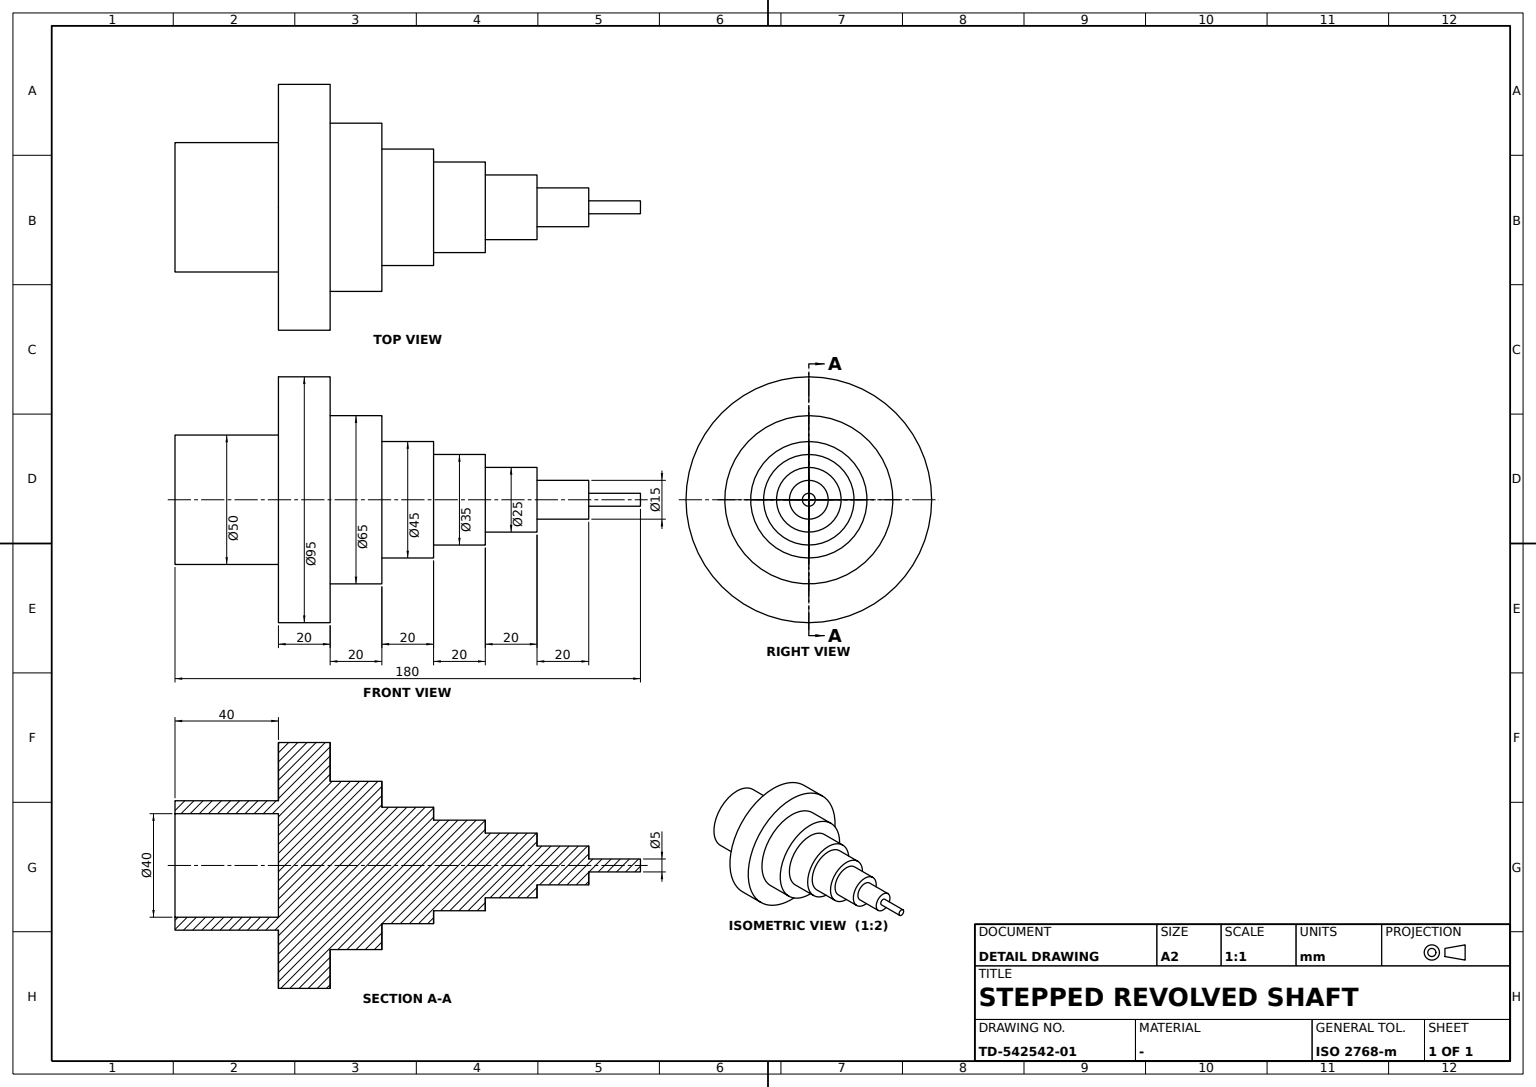
ISO-10303-21;
HEADER;
FILE_DESCRIPTION((''),'2;1');
FILE_NAME('','',(''),(''),'','','');
FILE_SCHEMA(('AUTOMOTIVE_DESIGN'));
ENDSEC;
DATA;
#1=APPLICATION_CONTEXT('');
#2=PRODUCT_CONTEXT('',#1,'mechanical');
#3=PRODUCT('','','',(#2));
#4=PRODUCT_DEFINITION_FORMATION('','',#3);
#5=PRODUCT_DEFINITION_CONTEXT('',#1,'design');
#6=PRODUCT_DEFINITION('','',#4,#5);
#7=PRODUCT_DEFINITION_SHAPE('','',#6);
#8=(LENGTH_UNIT()NAMED_UNIT(*)SI_UNIT(.MILLI.,.METRE.));
#9=(NAMED_UNIT(*)PLANE_ANGLE_UNIT()SI_UNIT($,.RADIAN.));
#10=(NAMED_UNIT(*)SI_UNIT($,.STERADIAN.)SOLID_ANGLE_UNIT());
#11=UNCERTAINTY_MEASURE_WITH_UNIT(LENGTH_MEASURE(0.005),#8,'distance_accuracy_value','');
#12=(GEOMETRIC_REPRESENTATION_CONTEXT(3)GLOBAL_UNCERTAINTY_ASSIGNED_CONTEXT((#11))GLOBAL_UNIT_ASSIGNED_CONTEXT((#8,#9,#10))REPRESENTATION_CONTEXT('',''));
#13=CARTESIAN_POINT('',(0.,140.,12.5));
#14=VERTEX_POINT('',#13);
#15=CARTESIAN_POINT('',(0.,140.,0.));
#16=DIRECTION('',(0.,1.,0.));
#17=DIRECTION('',(0.,0.,1.));
#18=AXIS2_PLACEMENT_3D('',#15,#16,#17);
#19=CIRCLE('',#18,12.5);
#20=EDGE_CURVE('',#14,#14,#19,.T.);
#21=ORIENTED_EDGE('',*,*,#20,.T.);
#22=EDGE_LOOP('',(#21));
#23=FACE_BOUND('',#22,.T.);
#24=CARTESIAN_POINT('',(0.,140.,7.5));
#25=VERTEX_POINT('',#24);
#26=CIRCLE('',#18,7.5);
#27=EDGE_CURVE('',#25,#25,#26,.T.);
#28=ORIENTED_EDGE('',*,*,#27,.F.);
#29=EDGE_LOOP('',(#28));
#30=FACE_BOUND('',#29,.T.);
#31=DIRECTION('',(1.,0.,0.));
#32=AXIS2_PLACEMENT_3D('',#13,#16,#31);
#33=PLANE('',#32);
#34=ADVANCED_FACE('',(#23,#30),#33,.T.);
#35=CARTESIAN_POINT('',(0.,40.,20.));
#36=VERTEX_POINT('',#35);
#37=CARTESIAN_POINT('',(0.,40.,0.));
#38=AXIS2_PLACEMENT_3D('',#37,#16,#17);
#39=CIRCLE('',#38,20.);
#40=EDGE_CURVE('',#36,#36,#39,.T.);
#41=ORIENTED_EDGE('',*,*,#40,.F.);
#42=EDGE_LOOP('',(#41));
#43=FACE_BOUND('',#42,.T.);
#44=CARTESIAN_POINT('',(0.,40.,25.));
#45=AXIS2_PLACEMENT_3D('',#44,#16,#31);
#46=PLANE('',#45);
#47=ADVANCED_FACE('',(#43),#46,.F.);
#48=CARTESIAN_POINT('',(0.,60.,32.5));
#49=VERTEX_POINT('',#48);
#50=CARTESIAN_POINT('',(0.,60.,0.));
#51=AXIS2_PLACEMENT_3D('',#50,#16,#17);
#52=CIRCLE('',#51,32.5);
#53=EDGE_CURVE('',#49,#49,#52,.T.);
#54=ORIENTED_EDGE('',*,*,#53,.F.);
#55=EDGE_LOOP('',(#54));
#56=FACE_BOUND('',#55,.T.);
#57=CARTESIAN_POINT('',(0.,60.,47.5));
#58=VERTEX_POINT('',#57);
#59=CIRCLE('',#51,47.5);
#60=EDGE_CURVE('',#58,#58,#59,.T.);
#61=ORIENTED_EDGE('',*,*,#60,.T.);
#62=EDGE_LOOP('',(#61));
#63=FACE_BOUND('',#62,.T.);
#64=AXIS2_PLACEMENT_3D('',#57,#16,#31);
#65=PLANE('',#64);
#66=ADVANCED_FACE('',(#56,#63),#65,.T.);
#67=CARTESIAN_POINT('',(0.,100.,17.5));
#68=VERTEX_POINT('',#67);
#69=CARTESIAN_POINT('',(0.,100.,0.));
#70=AXIS2_PLACEMENT_3D('',#69,#16,#17);
#71=CIRCLE('',#70,17.5);
#72=EDGE_CURVE('',#68,#68,#71,.T.);
#73=ORIENTED_EDGE('',*,*,#72,.T.);
#74=EDGE_LOOP('',(#73));
#75=FACE_BOUND('',#74,.T.);
#76=CARTESIAN_POINT('',(0.,120.,17.5));
#77=VERTEX_POINT('',#76);
#78=CARTESIAN_POINT('',(0.,120.,0.));
#79=AXIS2_PLACEMENT_3D('',#78,#16,#17);
#80=CIRCLE('',#79,17.5);
#81=EDGE_CURVE('',#77,#77,#80,.T.);
#82=ORIENTED_EDGE('',*,*,#81,.F.);
#83=EDGE_LOOP('',(#82));
#84=FACE_BOUND('',#83,.T.);
#85=CARTESIAN_POINT('',(0.,90.,0.));
#86=AXIS2_PLACEMENT_3D('',#85,#16,#31);
#87=CYLINDRICAL_SURFACE('',#86,17.5);
#88=ADVANCED_FACE('',(#75,#84),#87,.T.);
#89=ORIENTED_EDGE('',*,*,#60,.F.);
#90=EDGE_LOOP('',(#89));
#91=FACE_BOUND('',#90,.T.);
#92=CARTESIAN_POINT('',(0.,40.,47.5));
#93=VERTEX_POINT('',#92);
#94=CIRCLE('',#38,47.5);
#95=EDGE_CURVE('',#93,#93,#94,.T.);
#96=ORIENTED_EDGE('',*,*,#95,.T.);
#97=EDGE_LOOP('',(#96));
#98=FACE_BOUND('',#97,.T.);
#99=CYLINDRICAL_SURFACE('',#86,47.5);
#100=ADVANCED_FACE('',(#91,#98),#99,.T.);
#101=CARTESIAN_POINT('',(0.,100.,22.5));
#102=VERTEX_POINT('',#101);
#103=CIRCLE('',#70,22.5);
#104=EDGE_CURVE('',#102,#102,#103,.T.);
#105=ORIENTED_EDGE('',*,*,#104,.T.);
#106=EDGE_LOOP('',(#105));
#107=FACE_BOUND('',#106,.T.);
#108=ORIENTED_EDGE('',*,*,#72,.F.);
#109=EDGE_LOOP('',(#108));
#110=FACE_BOUND('',#109,.T.);
#111=AXIS2_PLACEMENT_3D('',#101,#16,#31);
#112=PLANE('',#111);
#113=ADVANCED_FACE('',(#107,#110),#112,.T.);
#114=CARTESIAN_POINT('',(0.,120.,12.5));
#115=VERTEX_POINT('',#114);
#116=CIRCLE('',#79,12.5);
#117=EDGE_CURVE('',#115,#115,#116,.T.);
#118=ORIENTED_EDGE('',*,*,#117,.F.);
#119=EDGE_LOOP('',(#118));
#120=FACE_BOUND('',#119,.T.);
#121=ORIENTED_EDGE('',*,*,#81,.T.);
#122=EDGE_LOOP('',(#121));
#123=FACE_BOUND('',#122,.T.);
#124=AXIS2_PLACEMENT_3D('',#76,#16,#31);
#125=PLANE('',#124);
#126=ADVANCED_FACE('',(#120,#123),#125,.T.);
#127=CARTESIAN_POINT('',(0.,160.,2.5));
#128=VERTEX_POINT('',#127);
#129=CARTESIAN_POINT('',(0.,160.,0.));
#130=AXIS2_PLACEMENT_3D('',#129,#16,#17);
#131=CIRCLE('',#130,2.5);
#132=EDGE_CURVE('',#128,#128,#131,.T.);
#133=ORIENTED_EDGE('',*,*,#132,.T.);
#134=EDGE_LOOP('',(#133));
#135=FACE_BOUND('',#134,.T.);
#136=CARTESIAN_POINT('',(0.,180.,2.5));
#137=VERTEX_POINT('',#136);
#138=CARTESIAN_POINT('',(0.,180.,0.));
#139=AXIS2_PLACEMENT_3D('',#138,#16,#17);
#140=CIRCLE('',#139,2.5);
#141=EDGE_CURVE('',#137,#137,#140,.T.);
#142=ORIENTED_EDGE('',*,*,#141,.F.);
#143=EDGE_LOOP('',(#142));
#144=FACE_BOUND('',#143,.T.);
#145=CYLINDRICAL_SURFACE('',#86,2.5);
#146=ADVANCED_FACE('',(#135,#144),#145,.T.);
#147=CARTESIAN_POINT('',(0.,160.,7.5));
#148=VERTEX_POINT('',#147);
#149=CIRCLE('',#130,7.5);
#150=EDGE_CURVE('',#148,#148,#149,.T.);
#151=ORIENTED_EDGE('',*,*,#150,.F.);
#152=EDGE_LOOP('',(#151));
#153=FACE_BOUND('',#152,.T.);
#154=ORIENTED_EDGE('',*,*,#27,.T.);
#155=EDGE_LOOP('',(#154));
#156=FACE_BOUND('',#155,.T.);
#157=CYLINDRICAL_SURFACE('',#86,7.5);
#158=ADVANCED_FACE('',(#153,#156),#157,.T.);
#159=ORIENTED_EDGE('',*,*,#104,.F.);
#160=EDGE_LOOP('',(#159));
#161=FACE_BOUND('',#160,.T.);
#162=CARTESIAN_POINT('',(0.,80.,22.5));
#163=VERTEX_POINT('',#162);
#164=CARTESIAN_POINT('',(0.,80.,0.));
#165=AXIS2_PLACEMENT_3D('',#164,#16,#17);
#166=CIRCLE('',#165,22.5);
#167=EDGE_CURVE('',#163,#163,#166,.T.);
#168=ORIENTED_EDGE('',*,*,#167,.T.);
#169=EDGE_LOOP('',(#168));
#170=FACE_BOUND('',#169,.T.);
#171=CYLINDRICAL_SURFACE('',#86,22.5);
#172=ADVANCED_FACE('',(#161,#170),#171,.T.);
#173=CARTESIAN_POINT('',(0.,0.,20.));
#174=VERTEX_POINT('',#173);
#175=CARTESIAN_POINT('',(0.,0.,0.));
#176=AXIS2_PLACEMENT_3D('',#175,#16,#17);
#177=CIRCLE('',#176,20.);
#178=EDGE_CURVE('',#174,#174,#177,.T.);
#179=ORIENTED_EDGE('',*,*,#178,.F.);
#180=EDGE_LOOP('',(#179));
#181=FACE_BOUND('',#180,.T.);
#182=ORIENTED_EDGE('',*,*,#40,.T.);
#183=EDGE_LOOP('',(#182));
#184=FACE_BOUND('',#183,.T.);
#185=CARTESIAN_POINT('',(0.,0.1,0.));
#186=AXIS2_PLACEMENT_3D('',#185,#16,#31);
#187=CYLINDRICAL_SURFACE('',#186,20.);
#188=ADVANCED_FACE('',(#181,#184),#187,.F.);
#189=CARTESIAN_POINT('',(0.,80.,32.5));
#190=VERTEX_POINT('',#189);
#191=CIRCLE('',#165,32.5);
#192=EDGE_CURVE('',#190,#190,#191,.T.);
#193=ORIENTED_EDGE('',*,*,#192,.T.);
#194=EDGE_LOOP('',(#193));
#195=FACE_BOUND('',#194,.T.);
#196=ORIENTED_EDGE('',*,*,#167,.F.);
#197=EDGE_LOOP('',(#196));
#198=FACE_BOUND('',#197,.T.);
#199=AXIS2_PLACEMENT_3D('',#189,#16,#31);
#200=PLANE('',#199);
#201=ADVANCED_FACE('',(#195,#198),#200,.T.);
#202=ORIENTED_EDGE('',*,*,#192,.F.);
#203=EDGE_LOOP('',(#202));
#204=FACE_BOUND('',#203,.T.);
#205=ORIENTED_EDGE('',*,*,#53,.T.);
#206=EDGE_LOOP('',(#205));
#207=FACE_BOUND('',#206,.T.);
#208=CYLINDRICAL_SURFACE('',#86,32.5);
#209=ADVANCED_FACE('',(#204,#207),#208,.T.);
#210=ORIENTED_EDGE('',*,*,#141,.T.);
#211=EDGE_LOOP('',(#210));
#212=FACE_BOUND('',#211,.T.);
#213=AXIS2_PLACEMENT_3D('',#136,#16,#31);
#214=PLANE('',#213);
#215=ADVANCED_FACE('',(#212),#214,.T.);
#216=ORIENTED_EDGE('',*,*,#178,.T.);
#217=EDGE_LOOP('',(#216));
#218=FACE_BOUND('',#217,.T.);
#219=CARTESIAN_POINT('',(0.,0.,25.));
#220=VERTEX_POINT('',#219);
#221=CIRCLE('',#176,25.);
#222=EDGE_CURVE('',#220,#220,#221,.T.);
#223=ORIENTED_EDGE('',*,*,#222,.F.);
#224=EDGE_LOOP('',(#223));
#225=FACE_BOUND('',#224,.T.);
#226=AXIS2_PLACEMENT_3D('',#175,#16,#31);
#227=PLANE('',#226);
#228=ADVANCED_FACE('',(#218,#225),#227,.F.);
#229=ORIENTED_EDGE('',*,*,#150,.T.);
#230=EDGE_LOOP('',(#229));
#231=FACE_BOUND('',#230,.T.);
#232=ORIENTED_EDGE('',*,*,#132,.F.);
#233=EDGE_LOOP('',(#232));
#234=FACE_BOUND('',#233,.T.);
#235=AXIS2_PLACEMENT_3D('',#147,#16,#31);
#236=PLANE('',#235);
#237=ADVANCED_FACE('',(#231,#234),#236,.T.);
#238=ORIENTED_EDGE('',*,*,#222,.T.);
#239=EDGE_LOOP('',(#238));
#240=FACE_BOUND('',#239,.T.);
#241=VERTEX_POINT('',#44);
#242=CIRCLE('',#38,25.);
#243=EDGE_CURVE('',#241,#241,#242,.T.);
#244=ORIENTED_EDGE('',*,*,#243,.F.);
#245=EDGE_LOOP('',(#244));
#246=FACE_BOUND('',#245,.T.);
#247=CYLINDRICAL_SURFACE('',#86,25.);
#248=ADVANCED_FACE('',(#240,#246),#247,.T.);
#249=ORIENTED_EDGE('',*,*,#20,.F.);
#250=EDGE_LOOP('',(#249));
#251=FACE_BOUND('',#250,.T.);
#252=ORIENTED_EDGE('',*,*,#117,.T.);
#253=EDGE_LOOP('',(#252));
#254=FACE_BOUND('',#253,.T.);
#255=CYLINDRICAL_SURFACE('',#86,12.5);
#256=ADVANCED_FACE('',(#251,#254),#255,.T.);
#257=ORIENTED_EDGE('',*,*,#243,.T.);
#258=EDGE_LOOP('',(#257));
#259=FACE_BOUND('',#258,.T.);
#260=ORIENTED_EDGE('',*,*,#95,.F.);
#261=EDGE_LOOP('',(#260));
#262=FACE_BOUND('',#261,.T.);
#263=ADVANCED_FACE('',(#259,#262),#46,.F.);
#264=CLOSED_SHELL('',(#34,#47,#66,#88,#100,#113,#126,#146,#158,#172,#188,#201,#209,#215,#228,#237,#248,#256,#263));
#265=MANIFOLD_SOLID_BREP('',#264);
#266=ADVANCED_BREP_SHAPE_REPRESENTATION('',(#265),#12);
#267=SHAPE_DEFINITION_REPRESENTATION(#7,#266);
ENDSEC;
END-ISO-10303-21;
